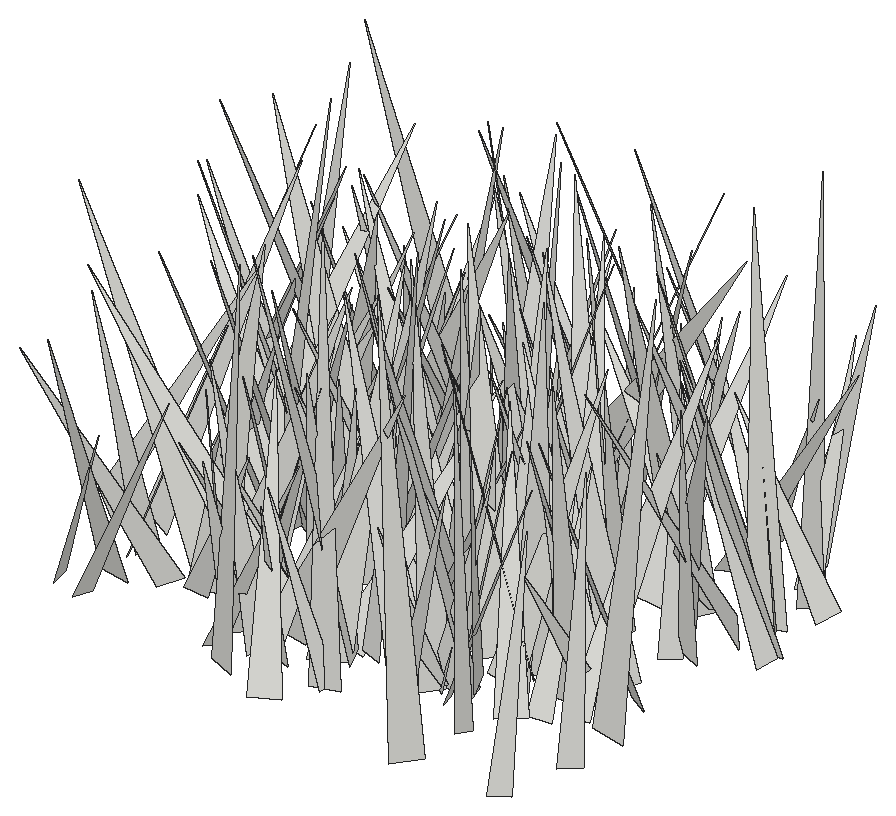
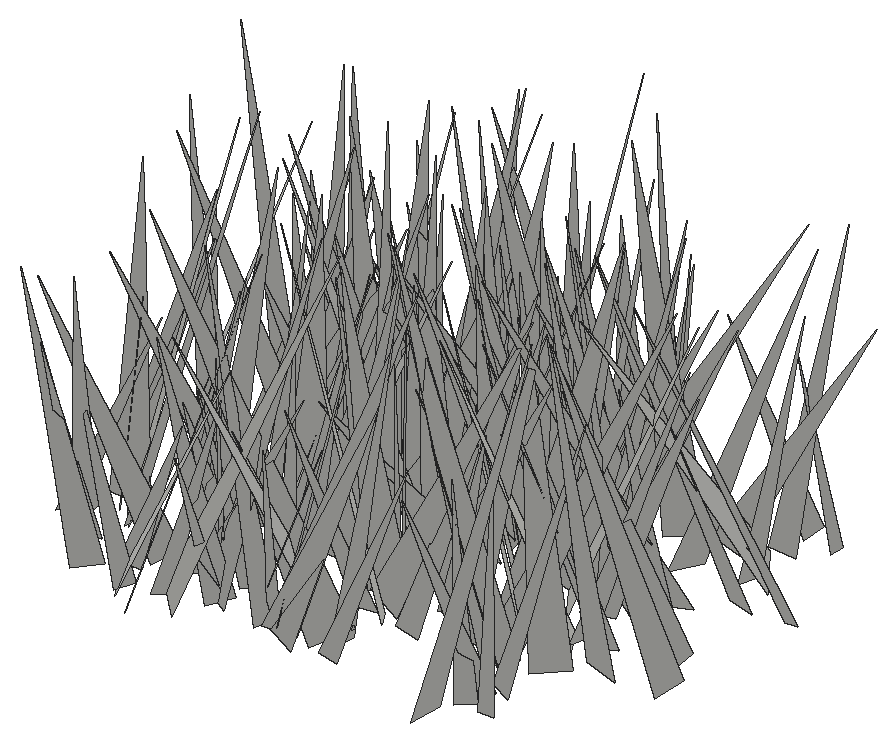
# SketchUp Ruby script. Lengths in inches.
U = 1.inch
M = Sketchup.active_model
def pt(a) = Geom::Point3d.new(a.map { |v| v * U })
def face(e, loops, mat)
  f = e.add_face(loops[0].map { |a| pt(a) })
  loops[1..].each { |l| e.add_face(l.map { |a| pt(a) }).erase! }
  f.material = f.back_material = mat if mat
  f
end
# faces: each face lists its corners as indices into pts; further lists are holes
def faces(e, pts, list, mat = nil) = list.each { |f| face(e, (f[0].is_a?(Array) ? f : [f]).map { |l| l.map { |i| pts[i] } }, mat) }
# xy, xz, yz: faces in a plane at the given z, y or x. An outline is a flat list of corners, or four numbers for a rectangle; further outlines are holes
def ring(l) = l.size == 4 ? [[l[0], l[1]], [l[2], l[1]], [l[2], l[3]], [l[0], l[3]]] : l.each_slice(2).to_a
def flat(e, list, mat, &to3) = list.each { |f| face(e, (f[0].is_a?(Array) ? f : [f]).map { |l| ring(l).map { |u, v| to3.(u, v) } }, mat) }
def xy(e, z, list, mat = nil) = flat(e, list, mat) { |x, y| [x, y, z] }
def xz(e, y, list, mat = nil) = flat(e, list, mat) { |x, z| [x, y, z] }
def yz(e, x, list, mat = nil) = flat(e, list, mat) { |y, z| [x, y, z] }
def lines(e, pts, list) = list.each { |a, b| e.add_line(pt(pts[a]), pt(pts[b])) }
# prism: a flat outline (further loops are holes) pulled along v
def prism(e, loops, v, mat = nil)
  f = face(e, loops, mat); d = Geom::Vector3d.new(v.map { |x| x * U })
  f.pushpull(f.normal.samedirection?(d) ? d.length : -d.length)
end
def box(e, o, s, mat = nil) = prism(e, [[o, [o[0] + s[0], o[1], o[2]], [o[0] + s[0], o[1] + s[1], o[2]], [o[0], o[1] + s[1], o[2]]]], [0, 0, s[2]], mat)
def at(x, y, z, deg = 0) = Geom::Transformation.translation(pt([x, y, z])) * Geom::Transformation.rotation(ORIGIN, Z_AXIS, deg.degrees)
def axes(o, x, y, z) = Geom::Transformation.new([*x, 0, *y, 0, *z, 0, *pt(o).to_a, 1])
def part(name) = M.definitions.add(name)
# library, detail: a bought-in or finely detailed component or shape, given as its bounding box
def library(name, o, s) = part(name).tap { |d| box(d.entities, o, s) }
def detail(e, o, s) = box(e.add_group.entities, o, s)
def put(e, d, t, mat = nil) = e.add_instance(d, t).tap { |i| i.material = mat if mat }
def group(e, t, mat = nil) = e.add_group.tap { |g| g.transformation = t; g.material = mat if mat }.entities
root = M.entities
c1 = part("fur_instance\#9")
p = [[0.8125,0,1.79],[0.67,-0.02,1.48],[0,-0.11,0],[0,0.11,0]]
faces(c1.entities,p,[[0,1,2,3]])
put(root,c1,axes([103.48,253.53,-27.1],[-0.9776,-5.25666,1.94415],[-5.10339,1.65068,1.89699],[2.31681,1.41798,4.99896]))
put(root,c1,axes([109.98,250.93,-27.1],[-4.30895,1.90574,0.59057],[1.67064,4.21479,-1.41144],[1.09067,1.07302,4.49519]))
put(root,c1,axes([98,253.64,-27.1],[-0.65259,-3.58567,0.77528],[-3.62638,0.74954,0.41412],[0.55447,0.682,3.62097]))
put(root,c1,axes([89.63,254.8125,-27.1],[-0.57876,-6.04691,0.53315],[-6.05695,0.61084,0.35302],[0.40347,0.49606,6.06428]))
put(root,c1,axes([99.22,251.23,-27.1],[-1.93628,5.55,0.46539],[5.55779,1.89356,0.54185],[-0.36056,-0.61659,5.85304]))
put(root,c1,axes([96.62,252.07,-27.1],[3.17531,6.56755,2.54139],[6.79761,-3.58673,0.77578],[-1.83954,-1.91744,7.25351]))
put(root,c1,axes([95.52,254.29,-27.1],[2.55514,-3.36467,0.69917],[-3.31318,-2.64324,-0.61213],[-0.91251,0.1757,4.18031]))
put(root,c1,axes([100.41,253.29,-27.1],[-3.8674,0.14725,0.40736],[0.1724,3.88071,0.23399],[0.39736,-0.25058,3.86312]))
put(root,c1,axes([105.92,250.83,-27.1],[-8.22184,1.12863,0.67504],[0.91948,7.98903,-2.15825],[0.94024,2.05661,8.01339]))
put(root,c1,axes([88.22,253.53,-27.1],[3.62066,0.28745,0.41277],[0.34104,-3.60783,-0.479],[-0.36973,-0.51296,3.60033]))
put(root,c1,axes([95.45,253.12,-27.1],[4.11337,-1.35782,0.42666],[-1.42017,-4.00175,0.95638],[-0.09392,1.04301,4.22479]))
put(root,c1,axes([95.85,253.41,-27.1],[-3.35833,-3.2337,1.73378],[-3.57177,3.41915,-0.54142],[0.83981,1.61055,4.63056]))
put(root,c1,axes([89.6,253.08,-27.1],[4.44559,-0.41699,0.42413],[-0.48383,-4.39553,0.74982],[-0.34594,0.78895,4.4017]))
put(root,c1,axes([96.93,253.87,-27.1],[-5.40914,1.11965,1.3835],[1.23539,5.5484,0.3398],[1.28121,-0.62292,5.51334]))
put(root,c1,axes([91.48,255.66,-27.1],[0.83306,-5.07313,1.39633],[-4.3947,-1.44829,-2.63999],[-2.89363,0.73905,4.41148]))
put(root,c1,axes([103.39,255.64,-27.1],[1.75124,-3.26229,0.83742],[-3.12175,-1.92651,-0.97669],[-1.26432,0.23809,3.57148]))
put(root,c1,axes([96.93,255.32,-27.1],[2.93254,-6.52755,1.0505],[-6.19008,-2.30697,2.94501],[2.32281,2.09313,6.52193]))
put(root,c1,axes([96.53,256,-27.1],[-0.29394,-4.28793,0.2812],[-4.0742,0.18848,-1.38464],[-1.36614,0.36048,4.06885]))
put(root,c1,axes([96.73,256.39,-27.1],[-3.34858,-4.98605,1.16696],[-4.83329,3.53804,1.24784],[1.69169,0.23891,5.87509]))
put(root,c1,axes([99.67,255.78,-27.1],[-7.3935,-3.44968,1.78048],[-3.41196,7.60131,0.55924],[1.85173,0.23234,8.13949]))
put(root,c1,axes([96.3,256.15,-27.1],[-7.10232,2.48969,0.17848],[2.39972,6.66255,2.55443],[-0.68683,-2.46683,7.07929]))
put(root,c1,axes([92.61,255.64,-27.1],[1.69765,-3.69471,0.41656],[-3.54176,-1.46758,1.41724],[1.13153,0.9496,3.81108]))
put(root,c1,axes([100.46,253.08,-27.1],[1.13757,8.04859,1.54719],[7.76789,-1.55698,2.3882],[-2.61411,-1.12413,7.76984]))
put(root,c1,axes([97.34,253.61,-27.1],[-2.89965,3.32427,1.06428],[2.78447,3.03733,-1.90073],[2.1048,0.5615,3.98069]))
put(root,c1,axes([110.67,254.03,-27.1],[-4.9436,1.78617,0.77223],[1.56135,4.89918,-1.33648],[1.16143,1.01666,5.08364]))
put(root,c1,axes([106.16,253.71,-27.1],[-6.18556,-0.57175,1.0735],[-0.94708,5.75521,-2.39186],[0.76312,2.5082,5.73298]))
put(root,c1,axes([104.51,256.58,-27.1],[-4.3896,-2.50757,2.34029],[-2.3133,4.97071,0.98703],[2.5325,0.19407,4.95805]))
put(root,c1,axes([102.49,255.31,-27.1],[-6.29408,3.56033,1.19684],[3.6784,6.31519,0.55815],[0.76008,-1.07993,7.20971]))
put(root,c1,axes([103.33,255.98,-27.1],[0.04539,-4.24616,1.86431],[-4.44886,0.48634,1.21602],[1.30888,1.80033,4.06857]))
put(root,c1,axes([95.48,255.65,-27.1],[5.08569,0.11573,0.95874],[0.07501,-5.17107,0.22632],[-0.96278,0.20845,5.08197]))
put(root,c1,axes([93.01,255.97,-27.1],[-2.73382,6.12597,3.74599],[6.6709,3.64992,-1.10045],[2.6569,-2.86083,6.61742]))
put(root,c1,axes([96.35,257.42,-27.1],[-3.41179,-1.77285,0.16017],[-1.67154,3.30984,1.02951],[0.61205,-0.84317,3.70451]))
put(root,c1,axes([96.98,257.43,-27.1],[3.24454,-4.71501,1.03025],[-4.7617,-3.32972,-0.24278],[-0.78672,0.70811,5.71834]))
put(root,c1,axes([89.28,257.09,-27.1],[-5.12264,0.34016,1.65759],[0.60899,5.30124,0.79415],[1.57874,-0.94118,5.07212]))
put(root,c1,axes([104.32,255.1,-27.1],[3.89284,1.77366,0.49192],[1.64576,-3.86945,0.92782],[-0.82421,0.65077,4.17603]))
put(root,c1,axes([104.79,256.03,-27.1],[-7.44301,-3.63877,0.95843],[-3.76282,7.20814,-1.85509],[0.01898,2.08796,8.0745]))
put(root,c1,axes([98.05,257.03,-27.1],[4.42383,-2.92058,1.2942],[-2.99041,-4.56361,-0.07677],[-1.12348,0.64702,5.30039]))
put(root,c1,axes([100.23,255.91,-27.1],[-1.46329,-3.87448,2.4887],[-4.52721,1.6881,-0.03379],[0.84239,2.34204,4.14146]))
put(root,c1,axes([108.59,258.29,-27.1],[2.63611,-2.6678,0.56163],[-2.26437,-2.5776,-1.61563],[-1.51829,-0.78771,3.38467]))
put(root,c1,axes([99.3,254.74,-27.1],[-5.55671,4.70477,2.20019],[4.40361,5.97611,-1.65743],[2.7539,-0.06297,7.08977]))
put(root,c1,axes([103.92,256.28,-27.1],[4.05853,2.67005,1.15678],[2.78357,-4.14094,-0.20805],[-0.84796,-0.81387,4.85361]))
put(root,c1,axes([107.83,257.65,-27.1],[0.14601,-6.62439,2.10053],[-6.94709,-0.08453,0.21629],[0.18059,2.1039,6.62247]))
put(root,c1,axes([106.84,255.52,-27.1],[-4.29612,3.71614,0.38084],[3.69784,4.31285,-0.36964],[0.52979,0.03157,5.66831]))
put(root,c1,axes([101.72,259.32,-27.1],[-1.16201,-7.65185,1.0654],[-7.72512,1.16361,-0.06847],[0.09162,1.06366,7.73928]))
put(root,c1,axes([91.57,257.77,-27.1],[-7.37091,1.53228,0.84327],[1.65266,7.29739,1.18581],[0.57246,-1.33774,7.43452]))
put(root,c1,axes([105.21,258.66,-27.1],[-4.80805,-4.95386,1.3489],[-5.02147,4.92244,0.17909],[1.0701,0.84054,6.90116]))
put(root,c1,axes([107.86,258.06,-27.1],[1.52237,-3.55739,1.37163],[-3.65271,-1.78416,-0.57315],[-1.09275,1.00785,3.82677]))
put(root,c1,axes([103.53,255.43,-27.1],[-7.58228,1.17889,0.51367],[1.00041,7.33787,-2.07353],[0.80796,1.97752,7.38791]))
put(root,c1,axes([103.68,255.49,-27.1],[3.73526,4.02595,0.93613],[3.5763,-3.78049,1.98866],[-2.07237,0.73241,5.11915]))
put(root,c1,axes([109.67,259.0625,-27.1],[-3.13069,-4.74867,0.6646],[-4.79451,3.11096,-0.35688],[0.06511,0.75154,5.67659]))
put(root,c1,axes([107.67,256.04,-27.1],[-0.4926,4.67354,0.05511],[4.67276,0.49124,0.10792],[-0.10156,-0.0661,4.69819]))
put(root,c1,axes([110.29,256.59,-27.1],[2.12447,7.8086,2.15105],[8.03257,-2.31646,0.47574],[-1.03873,-1.94278,8.07844]))
put(root,c1,axes([99.2,255.93,-27.1],[-0.72981,5.66267,0.18679],[5.27184,0.7477,-2.06932],[2.0757,0.09199,5.32132]))
put(root,c1,axes([95.5,259.64,-27.1],[-0.07367,-4.26522,0.50041],[-4.16979,0.19077,1.01214],[1.02732,0.46845,4.14405]))
put(root,c1,axes([105.45,258.42,-27.1],[1.282,-6.99581,3.06835],[-7.6361,-1.26107,0.31524],[-0.21483,3.07701,7.10532]))
put(root,c1,axes([105.08,257.34,-27.1],[0.03903,6.40601,1.64221],[6.43648,0.34027,-1.48032],[1.51842,-1.60705,6.23275]))
put(root,c1,axes([98.98,258.61,-27.1],[7.15031,1.42356,2.57616],[1.59453,-7.56218,-0.24693],[-2.47399,-0.75958,7.28646]))
put(root,c1,axes([108.72,256.875,-27.1],[-1.96871,3.37657,0.07437],[3.27614,1.93014,-0.90775],[0.82077,0.39482,3.80171]))
put(root,c1,axes([101.26,257.03,-27.1],[4.64309,0.99306,0.50279],[0.80416,-4.48393,1.43003],[-0.7696,1.30595,4.52764]))
put(root,c1,axes([100.41,258.9,-27.1],[-3.73947,1.85603,0.44676],[1.90802,3.6015,1.00834],[-0.06253,-1.10111,4.05114]))
put(root,c1,axes([96.15,259.74,-27.1],[4.14097,0.37336,0.37849],[0.46882,-3.96604,-1.21698],[-0.25072,-1.24957,3.97567]))
put(root,c1,axes([106.59,260.29,-27.1],[-1.84979,-4.95748,0.73449],[-4.97918,1.90688,0.3307],[0.56907,0.57009,5.281]))
put(root,c1,axes([95.66,259.7,-27.1],[0.8315,-3.67241,0.7269],[-3.73531,-0.86356,-0.09004],[-0.24991,0.6885,3.76429]))
put(root,c1,axes([95.33,260.29,-27.1],[0.2797,-5.08952,0.70223],[-5.01624,-0.11848,1.13926],[1.11073,0.74654,4.96825]))
put(root,c1,axes([108.11,258.43,-27.1],[-4.76226,4.46867,0.77555],[4.53262,4.64929,1.04363],[-0.16086,-1.29026,6.44663]))
put(root,c1,axes([93.45,259.64,-27.1],[-3.66042,-4.84933,0.70173],[-4.78346,3.34689,-1.82316],[-1.06154,1.63996,5.79575]))
put(root,c1,axes([102.76,258.57,-27.1],[-6.8831,0.44539,2.18741],[0.27023,7.20464,-0.61666],[2.21588,0.50489,6.86987]))
put(root,c1,axes([92.375,258.87,-27.1],[1.25839,-5.65908,2.69216],[-6.0262,-0.33916,2.10388],[1.71982,2.95233,5.40207]))
put(root,c1,axes([103.74,258.71,-27.1],[-6.05615,5.17907,2.30301],[5.46239,6.23254,0.34836],[1.51293,-1.77094,7.96105]))
put(root,c1,axes([102.32,259.55,-27.1],[2.05705,-3.40779,1.21765],[-3.60141,-2.06493,0.30505],[-0.3543,1.20424,3.9688]))
put(root,c1,axes([92.71,261.58,-27.1],[-2.90954,-6.16313,0.64564],[-6.10361,2.97343,0.8781],[1.07095,0.20243,6.75859]))
put(root,c1,axes([86.18,258.62,-27.1],[3.46284,5.45761,0.55951],[5.19477,-3.049,-2.40992],[1.76435,-1.73432,5.99742]))
put(root,c1,axes([98.26,261.55,-27.1],[-5.70608,-2.81682,0.48614],[-2.67601,5.6456,1.30244],[1.0049,-0.96065,6.22877]))
put(root,c1,axes([96.38,261.12,-27.1],[-4.22859,-0.79072,0.99748],[-0.41595,4.12901,1.5098],[1.20299,-1.35177,4.02824]))
put(root,c1,axes([94.06,261.47,-27.1],[-1.823,-5.96341,0.88128],[-5.94354,1.93183,0.77754],[1.00658,0.60664,6.18716]))
put(root,c1,axes([100.49,260.4,-27.1],[6.63287,-1.89646,1.66739],[-1.83678,-6.83922,-0.47211],[-1.73291,-0.0097,6.88248]))
put(root,c1,axes([105.97,256.74,-27.1],[-6.32088,1.55628,0.92222],[1.03646,5.86264,-2.78949],[1.48264,2.53644,5.88169]))
put(root,c1,axes([107.03,259.84,-27.1],[-1.92463,-5.23066,1.71698],[-5.26178,1.21283,-2.20335],[-1.6191,2.27625,5.1195]))
put(root,c1,axes([104.8125,258.3125,-27.1],[-1.18605,7.62635,1.82441],[7.84154,1.15487,0.27022],[0.00582,-1.84431,7.7133]))
put(root,c1,axes([93.46,259.13,-27.1],[0.89706,4.01856,0.51185],[4.05094,-0.89322,-0.08685],[-0.02607,-0.51851,4.11655]))
put(root,c1,axes([92.5,261.3125,-27.1],[6.03259,-1.06555,0.38284],[-1.02373,-6.01977,-0.62323],[-0.48366,-0.54868,6.09418]))
put(root,c1,axes([102.65,259.125,-27.1],[-4.5808,2.50643,0.71678],[2.42315,4.62824,-0.69815],[0.96142,0.27723,5.1748]))
put(root,c1,axes([88.34,258.75,-27.1],[3.15625,6.97995,0.87784],[7.00121,-3.02246,-1.14023],[0.68808,-1.26383,7.57506]))
put(root,c1,axes([108.56,259.56,-27.1],[-7.87651,1.28049,0.44694],[1.23259,7.85729,-0.78901],[0.56579,0.70864,7.94081]))
put(root,c1,axes([89.11,256.23,-27.1],[6.66219,5.05954,0.23915],[4.47229,-6.06129,3.64695],[-2.37798,2.77537,7.52884]))
put(root,c1,axes([98.6875,260.92,-27.1],[-2.55012,3.64542,1.48438],[3.93085,2.44958,0.73729],[0.20222,-1.64502,4.38733]))
put(root,c1,axes([97.36,259.76,-27.1],[5.64038,0.84844,0.8162],[0.68974,-5.61874,1.07421],[-0.95409,0.95384,5.60177]))
put(root,c1,axes([96.61,259.58,-27.1],[6.53232,-2.04401,3.08815],[-2.89411,-6.72439,1.67109],[-2.31057,2.64395,6.63752]))
put(root,c1,axes([103.83,262.45,-27.1],[-3.87501,-4.05549,0.17386],[-4.05477,3.85598,-0.42797],[-0.18982,0.42113,5.59281]))
put(root,c1,axes([95.58,260.34,-27.1],[6.99973,1.86447,1.44835],[1.77883,-7.14461,0.6004],[-1.55233,0.22015,7.21886]))
put(root,c1,axes([89,262.15,-27.1],[3.52002,-2.83902,0.00242],[-2.82378,-3.50072,0.47096],[0.29379,0.3681,4.49764]))
put(root,c1,axes([106.98,259.91,-27.1],[0.16958,6.97336,1.46095],[6.91324,0.19239,-1.72074],[1.72314,-1.45812,6.75984]))
put(root,c1,axes([97.67,260.74,-27.1],[4.97353,-2.18793,2.98402],[-2.79783,-5.49524,0.634],[-2.42149,1.85546,5.39639]))
put(root,c1,axes([103.84,261.0625,-27.1],[-5.54027,1.19429,0.93196],[1.15956,5.61711,-0.30487],[0.97482,0.10593,5.65933]))
put(root,c1,axes([109.23,265.23,-27.1],[-5.37416,-4.85351,0.14678],[-4.51514,5.07548,2.5125],[1.7865,-1.77274,6.79157]))
put(root,c1,axes([93.1,262.5,-27.1],[-5.86461,-3.9483,0.52207],[-3.9663,5.70596,-1.40208],[-0.36068,1.452,6.92942]))
put(root,c1,axes([106.74,265.04,-27.1],[-0.05965,-7.49908,0.31223],[-6.76708,0.1888,3.24163],[3.24657,0.25574,6.76251]))
put(root,c1,axes([101.02,261.12,-27.1],[6.96857,2.87265,0.80723],[2.85827,-7.01507,0.2896],[-0.85676,-0.03815,7.53188]))
put(root,c1,axes([103.38,263.72,-27.1],[-6.6748,0.96554,1.83268],[1.43583,6.61336,1.7452],[1.49311,-2.0433,6.51456]))
put(root,c1,axes([91.78,261.1,-27.1],[4.31651,6.80061,2.35568],[7.01576,-4.58865,0.3914],[-1.60519,-1.76799,8.04533]))
put(root,c1,axes([108.96,262.75,-27.1],[-1.48378,-4.80354,1.85374],[-5.06695,1.70492,0.36217],[0.91449,1.65264,5.01442]))
put(root,c1,axes([99.99,264.3125,-27.1],[7.80174,-0.94154,1.76979],[-0.49694,-7.7978,-1.95786],[-1.94209,-1.78708,7.61055]))
put(root,c1,axes([94.63,262.1,-27.1],[5.61379,-0.0924,1.25595],[-0.17391,-5.73971,0.3551],[-1.24727,0.38445,5.60331]))
put(root,c1,axes([95.93,261.86,-27.1],[-2.4957,-1.61977,2.11338],[-2.18018,2.90599,-0.34732],[1.52869,1.50005,2.95492]))
put(root,c1,axes([91.89,262.33,-27.1],[-4.33384,4.15795,0.46311],[4.09626,4.08164,1.68703],[-0.85069,-1.52868,5.76409]))
put(root,c1,axes([97.25,261.45,-27.1],[1.39427,3.92432,0.17719],[3.92808,-1.39069,-0.10895],[0.04345,-0.20342,4.16322]))
put(root,c1,axes([99.05,261.7,-27.1],[-3.57557,6.64036,0.56629],[6.42877,3.26724,2.27945],[-1.75672,-1.55901,7.1891]))
put(root,c1,axes([105.2,261.55,-27.1],[-2.95766,6.66869,1.17233],[6.76114,2.97762,0.11972],[0.36439,-1.12067,7.29416]))
put(root,c1,axes([90.14,260.2,-27.1],[0.04279,8.23701,0.26485],[7.98617,0.02394,-2.03491],[2.0346,-0.26721,7.98181]))
put(root,c1,axes([94.18,263.58,-27.1],[-5.61004,5.72169,2.32507],[6.16954,5.3361,1.75473],[0.28367,-2.89906,7.81865]))
put(root,c1,axes([104.67,263.98,-27.1],[-5.00716,-3.11226,0.75462],[-3.18598,4.98296,-0.58898],[0.32424,0.90067,5.86608]))
put(root,c1,axes([106.28,262.55,-27.1],[-7.03444,-1.19576,1.59787],[-1.52444,6.99776,-1.47438],[1.28808,1.75153,6.98136]))
put(root,c1,axes([91.1875,264.07,-27.1],[-6.42244,0.41118,0.57395],[0.45958,6.42194,0.54196],[0.53597,-0.57954,6.41273]))
put(root,c1,axes([100.18,260.97,-27.1],[-3.33289,3.23483,0.32122],[2.5841,2.91556,-2.549],[1.97223,1.64647,3.88264]))
put(root,c1,axes([111.12,264.71,-27.1],[-1.48365,-5.76059,1.44193],[-5.8771,1.21156,-1.20691],[-0.85046,1.67706,5.82486]))
put(root,c1,axes([98.6875,264.71,-27.1],[3.47548,2.68418,2.07766],[3.24177,-3.50628,-0.89294],[-1.00618,-2.02524,4.29959]))
put(root,c1,axes([89.91,263.98,-27.1],[2.31497,4.33574,1.17317],[4.28428,-1.73503,-2.04175],[1.34907,-1.93005,4.47091]))
put(root,c1,axes([111.43,264.24,-27.1],[-5.40823,0.65228,0.52882],[0.69912,5.40686,0.48075],[0.46513,-0.5426,5.42617]))
put(root,c1,axes([99.375,264.12,-27.1],[-2.0645,-2.99831,1.70133],[-3.28642,2.31061,0.08412],[1.04107,1.34824,3.63936]))
put(root,c1,axes([108.54,262.3,-27.1],[-4.64664,1.60589,0.29185],[1.45378,4.47236,-1.46283],[0.74202,1.29401,4.69365]))
put(root,c1,axes([87.43,263.23,-27.1],[6.02676,-0.13267,0.65935],[-0.25057,-5.95995,1.09109],[-0.62414,1.1116,5.92866]))
put(root,c1,axes([107.24,265.63,-27.1],[2.57242,-3.23839,0.522],[-3.12857,-2.6216,-0.84629],[-0.98573,-0.13048,4.04824]))
put(root,c1,axes([108.75,267.33,-27.1],[-6.83559,-3.49227,1.59422],[-2.83471,6.78714,2.71329],[2.5888,-1.7893,7.18049]))
put(root,c1,axes([103.24,264.5,-27.1],[-3.28307,2.60382,1.30489],[2.8552,3.26547,0.66758],[0.57484,-1.34832,4.13676]))
put(root,c1,axes([93.46,265.18,-27.1],[-3.35024,-7.10363,1.41562],[-6.97339,2.74138,-2.74705],[-1.95891,2.39017,7.35795]))
put(root,c1,axes([97.37,264.29,-27.1],[-4.10469,4.34568,0.4298],[4.19686,3.76273,2.03626],[-1.20665,-1.6956,5.62024]))
put(root,c1,axes([90.53,263.98,-27.1],[3.62784,4.7769,0.79864],[4.78599,-3.38301,-1.50576],[0.74217,-1.53438,5.80626]))
put(root,c1,axes([93.03,265.09,-27.1],[5.29628,3.42643,1.15131],[3.61426,-4.98862,-1.7797],[0.0553,-2.11891,6.05175]))
put(root,c1,axes([104.26,263.2,-27.1],[-3.06885,7.2619,1.47031],[7.40414,2.94663,0.90053],[-0.27521,-1.70206,7.83212]))
put(root,c1,axes([90.62,266.52,-27.1],[3.94338,-5.9757,0.15667],[-5.94055,-3.89659,0.90015],[0.66588,0.62564,7.10275]))
put(root,c1,axes([103.9375,264.59,-27.1],[-4.03311,-0.04964,1.55556],[-0.10181,4.31995,-0.1261],[1.55302,0.15428,4.03144]))
put(root,c1,axes([97.29,262.52,-27.1],[-7.34355,0.30763,3.29021],[-0.75169,7.65215,-2.39318],[3.21793,2.48952,6.94946]))
put(root,c1,axes([109.02,267.18,-27.1],[-5.87389,-5.06073,1.31002],[-4.91563,6.01764,1.20596],[1.77871,-0.08191,7.65893]))
put(root,c1,axes([86.6,264.9,-27.1],[6.73911,-0.51973,0.37006],[-0.5475,-6.72675,0.52311],[-0.32757,0.55072,6.73884]))
put(root,c1,axes([96,265.47,-27.1],[1.13242,-3.28388,1.61058],[-3.44754,-1.52145,-0.67814],[-1.2216,1.24962,3.40681]))
put(root,c1,axes([101.37,264.84,-27.1],[-2.35431,6.5098,1.98677],[6.74258,1.94391,1.62058],[-0.92858,-2.38982,6.73008]))
put(root,c1,axes([96.31,267.47,-27.1],[-1.09873,-5.30096,0.04279],[-5.29764,1.09638,-0.20521],[-0.19227,0.08352,5.40974]))
put(root,c1,axes([91.31,264.39,-27.1],[5.4364,3.24485,0.19999],[3.25087,-5.4295,-0.27539],[-0.03035,-0.33899,6.32516]))
put(root,c1,axes([94.55,266.56,-27.1],[0.42808,-6.23217,1.75974],[-6.34467,-0.7568,-1.13683],[-1.29687,1.64535,6.14254]))
put(root,c1,axes([98.25,266.35,-27.1],[-2.1287,-6.56011,1.58213],[-6.38568,1.42177,-2.69649],[-2.18201,2.23898,6.34786]))
put(root,c1,axes([104.99,267.58,-27.1],[0.47812,-7.3143,1.47747],[-7.45136,-0.54714,-0.29732],[-0.39895,1.45332,7.32388]))
put(root,c1,axes([92.34,267.17,-27.1],[1.4912,-7.63112,1.5604],[-7.07021,-0.65953,3.53123],[3.26816,2.05513,6.92734]))
put(root,c1,axes([100.98,263.82,-27.1],[3.07038,6.62387,1.59445],[6.28566,-3.42873,2.13997],[-2.62838,-0.46188,6.98022]))
put(root,c1,axes([97.57,267.24,-27.1],[6.19787,3.91116,1.13836],[4.069,-5.84754,-2.06304],[0.19042,-2.34857,7.0324]))
put(root,c1,axes([99.47,266.82,-27.1],[-5.53788,-5.2946,2.37412],[-5.70348,5.57065,-0.88067],[1.06751,2.29618,7.61087]))
put(root,c1,axes([89.26,265.43,-27.1],[1.99412,7.08431,1.8343],[7.27705,-2.12036,0.27805],[-0.77249,-1.68678,7.35436]))
put(root,c1,axes([109.78,266.13,-27.1],[-0.81741,7.52572,2.31704],[7.8363,0.54876,0.98214],[-0.77303,-2.39493,7.506]))
put(root,c1,axes([98.56,265.62,-27.1],[-2.23719,7.0676,1.63885],[7.20712,2.3619,-0.34736],[0.83319,-1.45336,7.40509]))
put(root,c1,axes([105.26,264.98,-27.1],[-1.51128,6.4389,0.97646],[6.11666,1.74753,-2.05657],[2.23592,-0.42848,6.28601]))
put(root,c1,axes([110.18,266.16,-27.1],[-4.46035,-2.40279,1.6408],[-2.85913,4.17643,-1.65628],[0.53948,2.26814,4.788]))
put(root,c1,axes([91.15,268.7,-27.1],[-2.16973,-4.86696,0.63571],[-4.9077,2.16207,-0.19771],[0.07681,0.6613,5.32503]))
put(root,c1,axes([107.52,265.52,-27.1],[-7.36083,-0.13148,0.37404],[-0.23398,7.05478,-2.12469],[0.32007,2.13349,7.04874]))
put(root,c1,axes([105.9375,265.77,-27.1],[-2.69846,2.82224,0.09608],[2.72603,2.63813,-0.93001],[0.73688,0.57546,3.79233]))
put(root,c1,axes([111.05,268,-27.1],[-4.33776,1.46199,0.55548],[1.55819,4.18055,1.16497],[0.13425,-1.28363,4.42678]))
put(root,c1,axes([100.25,269.65,-27.1],[-5.41835,-3.58553,1.38238],[-3.2455,5.54933,1.6725],[2.0576,-0.68883,6.27832]))
put(root,c1,axes([102.42,267.4375,-27.1],[-3.43885,-1.25141,0.28396],[-1.28081,3.29756,-0.97876],[-0.07859,1.01608,3.52615]))
put(root,c1,axes([91.88,267.81,-27.1],[3.27603,2.91205,0.73309],[2.99826,-3.11162,-1.03833],[0.1671,-1.26001,4.25844]))
put(root,c1,axes([102.64,268.4,-27.1],[0.8957,-3.44027,0.95903],[-3.38159,-0.49886,1.36875],[1.14894,1.21373,3.28089]))
put(root,c1,axes([103.05,269.78,-27.1],[-3.74984,-6.28849,1.24601],[-6.40364,3.74219,-0.38514],[0.30173,1.26879,7.3115]))
put(root,c1,axes([104.47,268.53,-27.1],[-4.30239,2.31555,0.00735],[2.25428,4.18495,1.12996],[-0.52922,-0.99839,4.75348]))
put(root,c1,axes([98.13,269.4,-27.1],[4.31656,-7.06636,0.27005],[-6.24466,-3.6606,4.0303],[3.31821,2.3034,7.23345]))
put(root,c1,axes([106.26,268.5,-27.1],[4.90095,-2.69617,0.00541],[-2.57457,-4.67657,1.67032],[0.80058,1.46597,5.33842]))
put(root,c1,axes([103.5,268.79,-27.1],[2.79577,3.11606,1.7882],[3.42019,-3.00212,-0.11591],[-1.09992,-1.41467,4.18482]))
put(root,c1,axes([100.33,267.43,-27.1],[3.37937,2.22818,0.23171],[2.15143,-3.34494,0.78826],[-0.62436,0.53406,3.97033]))
put(root,c1,axes([98.47,267.08,-27.1],[-0.0626,5.05917,0.30688],[5.04763,0.09003,-0.45456],[0.45914,-0.29998,5.03909]))
put(root,c1,axes([100.6,270.01,-27.1],[6.84395,0.46131,0.76105],[0.6015,-6.74756,-1.31919],[-0.65589,-1.3745,6.73144]))
put(root,c1,axes([97.61,269.51,-27.1],[5.36084,-0.19835,3.29768],[0.06393,-6.27827,-0.48156],[-3.30302,-0.44345,5.34285]))
put(root,c1,axes([91.51,270.17,-27.1],[1.83451,-3.56347,0.05806],[-3.52397,-1.80394,0.62811],[0.53227,0.33851,3.95843]))
put(root,c1,axes([90.5,270.3125,-27.1],[-0.97115,-4.17934,0.95629],[-4.09852,1.19278,1.05068],[1.25838,0.65947,4.16006]))
put(root,c1,axes([99.59,270.58,-27.1],[-2.75065,-6.97463,1.22589],[-6.99898,2.47729,-1.60986],[-1.07823,1.71227,7.32256]))
put(root,c1,axes([97.34,270.61,-27.1],[-0.13278,-3.81265,0.23397],[-3.74221,0.08288,-0.77308],[-0.76609,0.25594,3.73581]))
put(root,c1,axes([102.79,269.82,-27.1],[4.10289,-2.86128,0.97197],[-3.01034,-4.01302,0.89377],[-0.2636,1.29386,4.92156]))
put(root,c1,axes([104.27,270.86,-27.1],[-5.74525,-5.95088,0.61636],[-5.93253,5.55629,-1.65334],[-0.77329,1.58601,8.10478]))
put(root,c1,axes([104.72,270.65,-27.1],[-3.60372,1.36671,1.25031],[1.68423,3.55609,0.96723],[0.77106,-1.37995,3.73084]))
put(root,c1,axes([99.84,270.21,-27.1],[-3.57331,4.48467,0.98446],[4.4978,3.16833,1.89248],[-0.92266,-1.92337,5.41289]))
put(root,c1,axes([106.88,269.76,-27.1],[-1.92431,3.57441,0.40694],[3.46774,1.72017,1.28872],[-0.95749,-0.95373,3.84949]))
put(root,c1,axes([109.36,268.97,-27.1],[-0.62067,4.74172,0.56344],[4.77083,0.63973,-0.12835],[0.20124,-0.5417,4.78044]))
put(root,c1,axes([100.51,269.67,-27.1],[1.055,3.81063,1.04337],[3.83467,-1.24762,0.6792],[-0.95124,-0.80317,3.89521]))
put(root,c1,axes([99.24,268.35,-27.1],[5.73522,3.47371,0.17785],[3.39582,-5.66618,1.16354],[-0.75282,0.90483,6.60345]))
put(root,c1,axes([91.6,269.05,-27.1],[-0.33332,4.6985,0.41104],[4.65173,0.39553,-0.74898],[0.77866,-0.35159,4.65038]))
put(root,c1,axes([106.1,271.04,-27.1],[3.40491,-1.73217,0.1961],[-1.74293,-3.39081,0.31125],[-0.03288,0.3664,3.80749]))
put(root,c1,axes([105.3,271.75,-27.1],[-6.81995,-3.62088,0.84533],[-3.65528,6.85252,-0.13797],[0.68141,0.51893,7.72033]))
put(root,c1,axes([106.34,271.12,-27.1],[-4.80301,-2.64529,0.12183],[-2.62964,4.73476,-0.865],[-0.31202,0.81591,5.41463]))
put(root,c1,axes([92.15,271.625,-27.1],[-7.83608,-0.63477,1.59162],[-0.4911,7.96997,0.76075],[1.64165,-0.64574,7.82485]))
put(root,c1,axes([108,270.73,-27.1],[-1.7832,4.7887,2.83203],[5.02838,2.65983,-1.33139],[2.38064,-2.03113,4.93345]))
put(root,c1,axes([110.11,268.2,-27.1],[-7.67594,0.43258,1.18162],[-0.05572,7.18028,-2.99063],[1.25708,2.9597,7.0826]))
put(root,c1,axes([103.39,269.46,-27.1],[0.25291,3.93977,0.05992],[3.89833,-0.25892,0.57035],[-0.57304,-0.02262,3.90646]))
